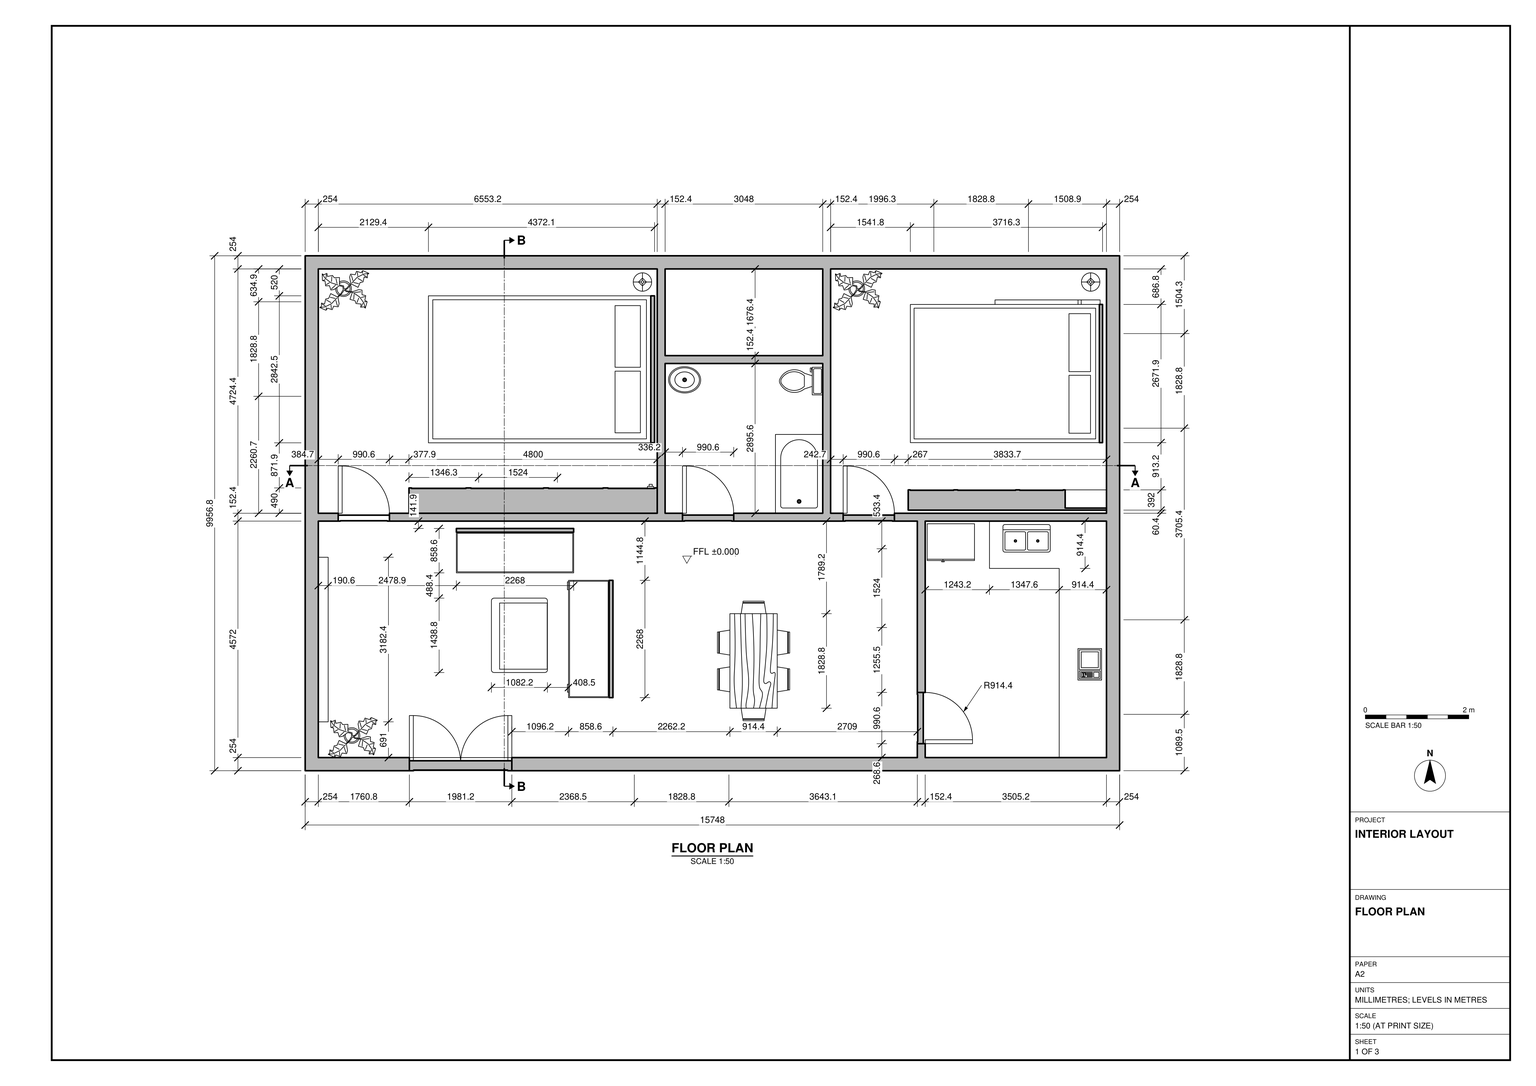
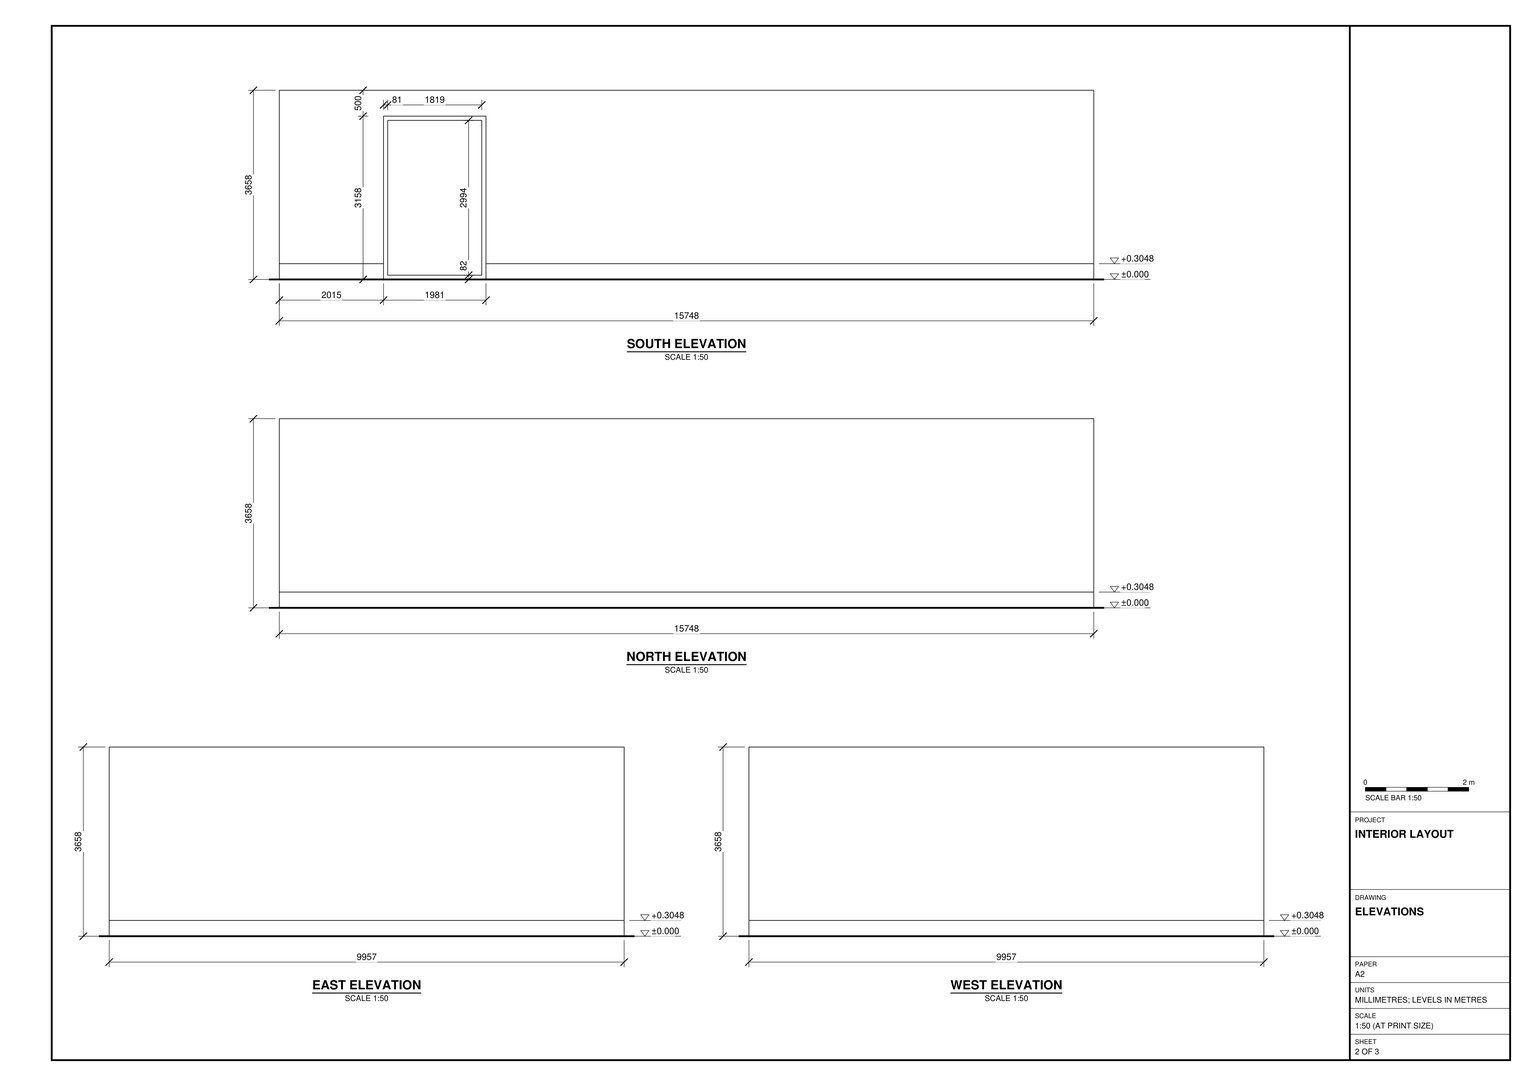
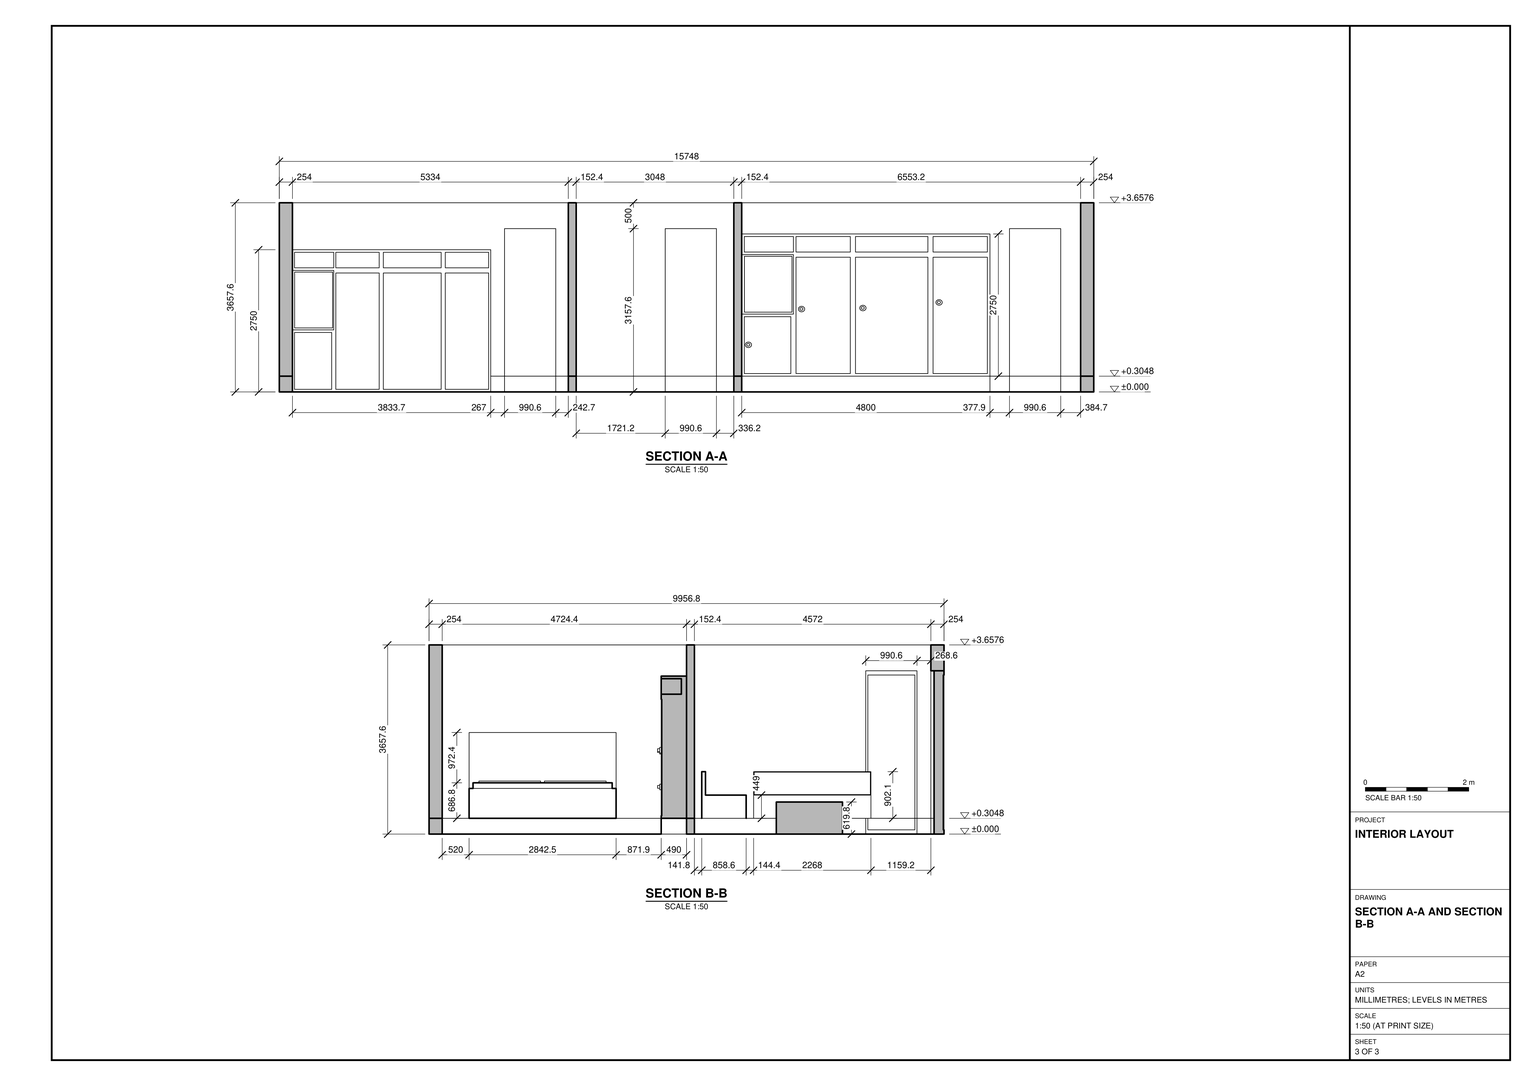
Build the interior in SketchUp using task_files/diagram_01.pdf. Work in millimetres. Use the floor plan to set out the rooms and the elevations and sections to establish heights. The rectangular shell measures 15748 mm east to west, 9956.8 mm north to south and 3657.6 mm high. Use a single ground-floor datum of 0 mm (±0.000). Model the floor base with the 304.8 mm base line shown in section, the 254 mm perimeter walls and the 152.4 mm partitions.

Place the bedrooms along the north side, with the bathroom between them and a separate enclosed space immediately north of the bathroom. Fit each bedroom with a bed and a built-in wardrobe along the south partition. Use section A-A for the wardrobe heights and front divisions, leaving room beside each wardrobe for the bedroom door. Place the basin, toilet and bathtub as shown in plan.

Set the double entrance door toward the west end of the south wall. Arrange the sofas and coffee table in the southwest living area, with the dining table and chairs between the seating and the enclosed southeast kitchen. Model the kitchen counter, double sink and appliances in their drawn positions. Decor and loose items such as plants, lamps and appliances may be any suitable library components.

Keep shell elements and individual furniture and joinery pieces in separate groups or components, and use components for repeated parts. Save one SketchUp model as output_files/furnished_two_bedroom_interior_with_built_in_wardrobes.skp.

# SketchUp Ruby script. Lengths in millimetres.
U = 1.mm
M = Sketchup.active_model
def pt(a) = Geom::Point3d.new(a.map { |v| v * U })
def face(e, loops, mat)
  f = e.add_face(loops[0].map { |a| pt(a) })
  loops[1..].each { |l| e.add_face(l.map { |a| pt(a) }).erase! }
  f.material = f.back_material = mat if mat
  f
end
# faces: each face lists its corners as indices into pts; further lists are holes
def faces(e, pts, list, mat = nil) = list.each { |f| face(e, (f[0].is_a?(Array) ? f : [f]).map { |l| l.map { |i| pts[i] } }, mat) }
# xy, xz, yz: faces in a plane at the given z, y or x. An outline is a flat list of corners, or four numbers for a rectangle; further outlines are holes
def ring(l) = l.size == 4 ? [[l[0], l[1]], [l[2], l[1]], [l[2], l[3]], [l[0], l[3]]] : l.each_slice(2).to_a
def flat(e, list, mat, &to3) = list.each { |f| face(e, (f[0].is_a?(Array) ? f : [f]).map { |l| ring(l).map { |u, v| to3.(u, v) } }, mat) }
def xy(e, z, list, mat = nil) = flat(e, list, mat) { |x, y| [x, y, z] }
def xz(e, y, list, mat = nil) = flat(e, list, mat) { |x, z| [x, y, z] }
def yz(e, x, list, mat = nil) = flat(e, list, mat) { |y, z| [x, y, z] }
def lines(e, pts, list) = list.each { |a, b| e.add_line(pt(pts[a]), pt(pts[b])) }
# prism: a flat outline (further loops are holes) pulled along v
def prism(e, loops, v, mat = nil)
  f = face(e, loops, mat); d = Geom::Vector3d.new(v.map { |x| x * U })
  f.pushpull(f.normal.samedirection?(d) ? d.length : -d.length)
end
def box(e, o, s, mat = nil) = prism(e, [[o, [o[0] + s[0], o[1], o[2]], [o[0] + s[0], o[1] + s[1], o[2]], [o[0], o[1] + s[1], o[2]]]], [0, 0, s[2]], mat)
def at(x, y, z, deg = 0) = Geom::Transformation.translation(pt([x, y, z])) * Geom::Transformation.rotation(ORIGIN, Z_AXIS, deg.degrees)
def axes(o, x, y, z) = Geom::Transformation.new([*x, 0, *y, 0, *z, 0, *pt(o).to_a, 1])
def part(name) = M.definitions.add(name)
# library, detail: a bought-in or finely detailed component or shape, given as its bounding box
def library(name, o, s) = part(name).tap { |d| box(d.entities, o, s) }
def detail(e, o, s) = box(e.add_group.entities, o, s)
def put(e, d, t, mat = nil) = e.add_instance(d, t).tap { |i| i.material = mat if mat }
def group(e, t, mat = nil) = e.add_group.tap { |g| g.transformation = t; g.material = mat if mat }.entities
root = M.entities
M.materials.add("[Carpet Pattern Squares Multi]").color = [138, 129, 101]
M.materials.add("[Color M08]").color = [30, 30, 30]
M.materials.add("[Color M09]").color = [0, 0, 0]
M.materials.add("[Leather Blue]").color = [45, 57, 74]
M.materials.add("[Mirror 02]").color = [229, 229, 229]
M.materials.add("[Translucent Glass Gray]").color = [128, 128, 128]
M.materials["[Translucent Glass Gray]"].alpha = 0.5
M.materials.add("[Wood Cherry Original]").color = [152, 86, 42]
M.materials.add("[Wood Veneer 01]").color = [120, 70, 37]
c1 = part("Framed panel")
xy(c1.entities,0,[[0,0,3940,620]],"[Wood Veneer 01]")
xy(c1.entities,161.4,[[161.4,0,3778.6,40]],"[Wood Veneer 01]")
xy(c1.entities,6068.6,[[161.4,0,3778.6,40]],"[Wood Veneer 01]")
xy(c1.entities,6230,[[0,0,3940,620]],"[Wood Veneer 01]")
xz(c1.entities,0,[[[0,0,3940,6230],[161.4,161.4,3778.6,6068.6]]],"[Wood Veneer 01]")
xz(c1.entities,40,[[161.4,161.4,3778.6,6068.6]],"[Wood Veneer 01]")
xz(c1.entities,620,[[0,0,3940,6230]],"[Wood Veneer 01]")
yz(c1.entities,0,[[0,0,620,6230]],"[Wood Veneer 01]")
yz(c1.entities,161.4,[[0,161.4,40,6068.6]],"[Wood Veneer 01]")
yz(c1.entities,3778.6,[[0,161.4,40,6068.6]],"[Wood Veneer 01]")
yz(c1.entities,3940,[[0,0,620,6230]],"[Wood Veneer 01]")
c2 = part("Component\#1")
xy(c2.entities,0,[[320,0,237.2,10.9,160,42.9,93.7,93.7,42.9,160,10.9,237.2,0,320,10.9,402.8,42.9,480,93.7,546.3,160,597.1,237.2,629.1,320,640,402.8,629.1,480,597.1,546.3,546.3,597.1,480,629.1,402.8,640,320,629.1,237.2,597.1,160,546.3,93.7,480,42.9,402.8,10.9]])
xy(c2.entities,230,[[[320,0,402.8,10.9,480,42.9,546.3,93.7,597.1,160,629.1,237.2,640,320,629.1,402.8,597.1,480,546.3,546.3,480,597.1,402.8,629.1,320,640,237.2,629.1,160,597.1,93.7,546.3,42.9,480,10.9,402.8,0,320,10.9,237.2,42.9,160,93.7,93.7,160,42.9,237.2,10.9],[322.3,149.9,281.5,158.6,244.3,177.6,213.2,205.6,190.5,240.7,177.6,280.4,175.5,322.1,184.2,363,203.2,400.2,231.2,431.2,266.2,453.9,305.9,466.8,347.7,468.9,388.5,460.2,425.7,441.2,456.7,413.2,479.5,378.2,492.3,338.5,494.5,296.8,485.8,255.9,466.8,218.7,438.8,187.7,403.8,165,364,152.1]]])
xy(c2.entities,470,[[322.3,149.9,364,152.1,403.8,165,438.8,187.7,466.8,218.7,485.8,255.9,494.5,296.8,492.3,338.5,479.5,378.2,456.7,413.2,425.7,441.2,388.5,460.2,347.7,468.9,305.9,466.8,266.2,453.9,231.2,431.2,203.2,400.2,184.2,363,175.5,322.1,177.6,280.4,190.5,240.7,213.2,205.6,244.3,177.6,281.5,158.6]])
p = [[237.2,10.9,0],[320,0,0],[320,0,230],[237.2,10.9,230],[402.8,10.9,0],[402.8,10.9,230],
  [160,42.9,0],[160,42.9,230],[480,42.9,0],[480,42.9,230],[93.7,93.7,0],[93.7,93.7,230],
  [546.3,93.7,0],[546.3,93.7,230],[42.9,160,0],[42.9,160,230],[597.1,160,0],[597.1,160,230],
  [10.9,237.2,0],[10.9,237.2,230],[629.1,237.2,0],[629.1,237.2,230],[0,320,0],[0,320,230],
  [640,320,0],[640,320,230],[10.9,402.8,0],[10.9,402.8,230],[629.1,402.8,0],[629.1,402.8,230],
  [42.9,480,0],[42.9,480,230],[597.1,480,0],[597.1,480,230],[93.7,546.3,0],[93.7,546.3,230],
  [546.3,546.3,0],[546.3,546.3,230],[160,597.1,0],[160,597.1,230],[480,597.1,0],[480,597.1,230],
  [237.2,629.1,0],[237.2,629.1,230],[402.8,629.1,0],[402.8,629.1,230],[320,640,0],[320,640,230],
  [281.5,158.6,230],[322.3,149.9,230],[322.3,149.9,470],[281.5,158.6,470],[364,152.1,230],[364,152.1,470],
  [403.8,165,230],[403.8,165,470],[244.3,177.6,230],[244.3,177.6,470],[438.8,187.7,230],[438.8,187.7,470],
  [213.2,205.6,230],[213.2,205.6,470],[466.8,218.7,230],[466.8,218.7,470],[190.5,240.7,230],[190.5,240.7,470],
  [485.8,255.9,230],[485.8,255.9,470],[177.6,280.4,230],[177.6,280.4,470],[494.5,296.8,230],[494.5,296.8,470],
  [175.5,322.1,230],[175.5,322.1,470],[492.3,338.5,230],[492.3,338.5,470],[184.2,363,230],[184.2,363,470],
  [479.5,378.2,230],[479.5,378.2,470],[203.2,400.2,230],[203.2,400.2,470],[456.7,413.2,230],[456.7,413.2,470],
  [231.2,431.2,230],[231.2,431.2,470],[425.7,441.2,230],[425.7,441.2,470],[266.2,453.9,230],[266.2,453.9,470],
  [388.5,460.2,230],[388.5,460.2,470],[305.9,466.8,230],[305.9,466.8,470],[347.7,468.9,230],[347.7,468.9,470]]
faces(c2.entities,p,[[0,1,2,3],[1,4,5,2],[6,0,3,7],[4,8,9,5],[10,6,7,11],[8,12,13,9],[14,10,11,15],[12,16,17,13],
  [18,14,15,19],[16,20,21,17],[22,18,19,23],[20,24,25,21],[26,22,23,27],[24,28,29,25],[30,26,27,31],[28,32,33,29],
  [34,30,31,35],[32,36,37,33],[38,34,35,39],[36,40,41,37],[42,38,39,43],[40,44,45,41],[46,42,43,47],[44,46,47,45],
  [48,49,50,51],[49,52,53,50],[52,54,55,53],[56,48,51,57],[54,58,59,55],[60,56,57,61],[58,62,63,59],[64,60,61,65],
  [62,66,67,63],[68,64,65,69],[66,70,71,67],[72,68,69,73],[70,74,75,71],[76,72,73,77],[74,78,79,75],[80,76,77,81],
  [78,82,83,79],[84,80,81,85],[82,86,87,83],[88,84,85,89],[86,90,91,87],[92,88,89,93],[90,94,95,91],[94,92,93,95]])
c3 = part("Bed frame")
xy(c3.entities,0,[[0,0,5267.6,3790]],"[Wood Veneer 01]")
xy(c3.entities,850,[[[0,0,5180,3790],[101.4,101.4,5078.6,3688.6]]],"[Wood Veneer 01]")
xy(c3.entities,1010,[[[101.4,101.4,5078.6,3688.6],[4347.5,257.5,4937.5,1847.5],[4347.5,1947.5,4937.5,3537.5]]],"[Leather Blue]")
xy(c3.entities,1060,[[4347.5,257.5,4937.5,1847.5],[4347.5,1947.5,4937.5,3537.5]])
xy(c3.entities,2440,[[5180,0,5267.6,3790]],"[Wood Veneer 01]")
xz(c3.entities,0,[[0,0,5267.6,0,5267.6,2440,5180,2440,5180,850,0,850]],"[Wood Veneer 01]")
xz(c3.entities,101.4,[[101.4,850,5078.6,1010]],"[Leather Blue]")
xz(c3.entities,257.5,[[4347.5,1010,4937.5,1060]])
xz(c3.entities,1847.5,[[4347.5,1010,4937.5,1060]])
xz(c3.entities,1947.5,[[4347.5,1010,4937.5,1060]])
xz(c3.entities,3537.5,[[4347.5,1010,4937.5,1060]])
xz(c3.entities,3688.6,[[101.4,850,5078.6,1010]],"[Leather Blue]")
xz(c3.entities,3790,[[0,0,0,850,5180,850,5180,2440,5267.6,2440,5267.6,0]],"[Wood Veneer 01]")
yz(c3.entities,0,[[0,0,3790,850]],"[Wood Veneer 01]")
yz(c3.entities,101.4,[[101.4,850,3688.6,1010]],"[Leather Blue]")
yz(c3.entities,4347.5,[[257.5,1010,1847.5,1060],[1947.5,1010,3537.5,1060]])
yz(c3.entities,4937.5,[[257.5,1010,1847.5,1060],[1947.5,1010,3537.5,1060]])
yz(c3.entities,5078.6,[[101.4,850,3688.6,1010]],"[Leather Blue]")
yz(c3.entities,5180,[[0,850,3790,2440]],"[Wood Veneer 01]")
yz(c3.entities,5267.6,[[0,0,3790,2440]],"[Wood Veneer 01]")
c4 = part("Component\#3")
xy(c4.entities,1000,[[[0,0,4320,1310],[33.6,33.6,4286.4,1276.4]],[33.6,33.6,4286.4,1276.4]])
xy(c4.entities,2010,[[0,1310,4320,1430]])
xz(c4.entities,0,[[0,0,4320,1000]])
xz(c4.entities,1310,[[[0,1000,4320,2010],[21.1,1021.1,4298.9,1988.9]],[21.1,1021.1,4298.9,1988.9]])
xz(c4.entities,1430,[[0,0,4320,2010]])
yz(c4.entities,0,[[0,0,0,1000,1310,1000,1310,2010,1430,2010,1430,0]])
yz(c4.entities,4320,[[0,0,1430,0,1430,2010,1310,2010,1310,1000,0,1000]])
c5 = library("floor plan.dwg",[0,0,0],[15748,9956.8,0.1])
c6 = part("Built-in wardrobe")
xy(c6.entities,304.8,[[2007.2,4978.4,6807.2,5468.4]])
xy(c6.entities,354.8,[[2057.2,5458.4,3107.2,5468.4],[3207.2,5458.4,4607.2,5468.4],[4707.2,5458.4,5757.2,5468.4],[5857.2,5458.4,6757.2,5468.4]],"[Wood Cherry Original]")
xy(c6.entities,1454.8,[[5857.2,5458.4,6757.2,5468.4]])
xy(c6.entities,1504.8,[[5807.2,5028.4,6807.2,5468.4]],"[Wood Cherry Original]")
xy(c6.entities,1542.2,[[5834.9,4988.4,6754.9,5028.4]],"[Color M09]")
xy(c6.entities,2604.8,[[2057.2,5458.4,3107.2,5468.4],[3207.2,5458.4,4607.2,5468.4],[4707.2,5458.4,5757.2,5468.4]],"[Wood Cherry Original]")
xy(c6.entities,2622.2,[[5834.9,4988.4,6754.9,5028.4]],"[Color M09]")
xy(c6.entities,2654.8,[[5807.2,5028.4,6807.2,5468.4]],"[Wood Cherry Original]")
xy(c6.entities,2704.8,[[2057.2,5078.4,3107.2,5468.4],[3207.2,5078.4,4607.2,5468.4],[4707.2,5078.4,5757.2,5468.4],[5807.2,5078.4,6757.2,5468.4]])
xy(c6.entities,3004.8,[[2057.2,5078.4,3107.2,5468.4],[3207.2,5078.4,4607.2,5468.4],[4707.2,5078.4,5757.2,5468.4],[5807.2,5078.4,6757.2,5468.4]])
xy(c6.entities,3054.8,[[2007.2,4978.4,6807.2,5468.4]],"[Wood Cherry Original]")
xz(c6.entities,4978.4,[[2007.2,304.8,6807.2,3054.8]])
xz(c6.entities,4988.4,[[5834.9,1542.2,6754.9,2622.2]],"[Mirror 02]")
xz(c6.entities,5028.4,[[[5807.2,1504.8,6807.2,2654.8],[5834.9,1542.2,6754.9,2622.2]]],"[Color M09]")
xz(c6.entities,5078.4,[[2057.2,2704.8,3107.2,3004.8],[3207.2,2704.8,4607.2,3004.8],[4707.2,2704.8,5757.2,3004.8],[5807.2,2704.8,6757.2,3004.8]])
xz(c6.entities,5458.4,[[2057.2,354.8,3107.2,2604.8],[3207.2,354.8,4607.2,2604.8],[4707.2,354.8,5757.2,2604.8],[5857.2,354.8,6757.2,1454.8]],"[Wood Cherry Original]")
xz(c6.entities,5468.4,[[2057.2,2704.8,3107.2,3004.8],[3207.2,2704.8,4607.2,3004.8],[4707.2,2704.8,5757.2,3004.8],[5807.2,2704.8,6757.2,3004.8]],"[Translucent Glass Gray]")
xz(c6.entities,5468.4,[[[2007.2,304.8,2007.2,3054.8,6807.2,3054.8,6807.2,2654.8,5807.2,2654.8,5807.2,1504.8,6807.2,1504.8,6807.2,304.8],[3207.2,354.8,4607.2,2604.8],[2057.2,354.8,3107.2,2604.8],[4707.2,354.8,5757.2,2604.8],[5857.2,354.8,6757.2,1454.8],[3207.2,2704.8,4607.2,3004.8],[2057.2,2704.8,3107.2,3004.8],[4707.2,2704.8,5757.2,3004.8],[5807.2,2704.8,6757.2,3004.8]]],"[Wood Cherry Original]")
yz(c6.entities,2007.2,[[4978.4,304.8,5468.4,3054.8]],"[Wood Cherry Original]")
yz(c6.entities,2057.2,[[5458.4,354.8,5468.4,2604.8]],"[Wood Cherry Original]")
yz(c6.entities,3107.2,[[5078.4,2704.8,5468.4,3004.8]])
yz(c6.entities,3107.2,[[5458.4,354.8,5468.4,2604.8]],"[Wood Cherry Original]")
yz(c6.entities,3207.2,[[5078.4,2704.8,5468.4,3004.8]])
yz(c6.entities,3207.2,[[5458.4,354.8,5468.4,2604.8]],"[Wood Cherry Original]")
yz(c6.entities,4607.2,[[5078.4,2704.8,5468.4,3004.8]])
yz(c6.entities,4607.2,[[5458.4,354.8,5468.4,2604.8]],"[Wood Cherry Original]")
yz(c6.entities,4707.2,[[5078.4,2704.8,5468.4,3004.8]])
yz(c6.entities,4707.2,[[5458.4,354.8,5468.4,2604.8]],"[Wood Cherry Original]")
yz(c6.entities,5757.2,[[5458.4,354.8,5468.4,1504.8],[5078.4,2704.8,5468.4,3004.8]])
yz(c6.entities,5757.2,[[5458.4,1504.8,5468.4,2604.8]],"[Wood Cherry Original]")
yz(c6.entities,5807.2,[[5078.4,2704.8,5468.4,3004.8]])
yz(c6.entities,5807.2,[[5028.4,1504.8,5468.4,2654.8]],"[Wood Cherry Original]")
yz(c6.entities,5834.9,[[4988.4,1542.2,5028.4,2622.2]],"[Color M09]")
yz(c6.entities,5857.2,[[5458.4,354.8,5468.4,1454.8]],"[Wood Cherry Original]")
yz(c6.entities,6754.9,[[4988.4,1542.2,5028.4,2622.2]],"[Color M09]")
yz(c6.entities,6757.2,[[5458.4,354.8,5468.4,1454.8],[5078.4,2704.8,5468.4,3004.8]])
yz(c6.entities,6807.2,[[4978.4,304.8,4978.4,3054.8,5468.4,3054.8,5468.4,2654.8,5028.4,2654.8,5028.4,1504.8,5468.4,1504.8,5468.4,304.8]])
c7 = part("Two-bedroom interior")
put(c7.entities,c2,axes([4983.2,6404.2,1676],[0.19072,0,0],[0,0,-0.1675],[0,0.17,0]),"[Color M08]")
put(c7.entities,c2,axes([3510.2,6404.2,1784.6],[0.19072,0,0],[0,0,-0.1675],[0,0.17,0]),"[Color M08]")
put(c7.entities,c2,axes([7197,6404.2,964.7],[0.19072,0,0],[0,0,-0.1675],[0,0.17,0]),"[Color M08]")
put(c7.entities,c3,axes([2963.3,7286.1,304.8],[0.83,0,0],[0,0.75,0],[0,0,0.68]))
put(c7.entities,c4,axes([3503.4,4771.4,304.8],[0.525,0,0],[0,0.6004,0],[0,0,0.4488]),"[Wood Cherry Original]")
put(c7.entities,c3,axes([12281.8,7289.9,0],[0.7055,0,0],[0,0.705,0],[0,0,0.68]))
put(c7.entities,c5,at(579.9,945.8,304.8))
put(c7.entities,c6,axes([10637.1,2001.9,-304.8],[0.79869,0,0],[0,0.8,0],[0,0,1]))
put(c7.entities,c4,axes([5672.1,4627,304.8],[0,-0.525,0],[0.6004,0,0],[0,0,0.4488]),"[Wood Cherry Original]")
put(c7.entities,c2,axes([6169.2,6404.3,1656.1],[0.19072,0,0],[0,0,-0.1675],[0,0.17,0]),"[Color M08]")
g1 = group(c7.entities,at(579.9,945.8,0))
xy(g1,0,[[0,0,0,9956.8,15748,9956.8,15748,0,3996,0,3996,254,15494,254,15494,9702.8,254,9702.8,254,254,2014.8,254,2014.8,0],[2014.8,0,3996,254],[254,254,11836.4,254,11836.4,522.6,11988.8,522.6,11988.8,254,15494,254,15494,4826,11988.8,4826,11988.8,1513.2,11836.4,1513.2,11836.4,4826,11393.3,4826,11393.3,4978.4,15494,4978.4,15494,9702.8,10160,9702.8,10160,4978.4,10402.7,4978.4,10402.7,4826,8286.4,4826,8286.4,4978.4,10007.6,4978.4,10007.6,7874,6959.6,7874,6959.6,4978.4,7295.8,4978.4,7295.8,4826,1629.3,4826,1629.3,4978.4,2007.2,4978.4,2007.2,5468.4,6807.2,5468.4,6807.2,9702.8,254,9702.8,254,4978.4,638.7,4978.4,638.7,4826,254,4826],[11836.4,254,11988.8,522.6],[11836.4,1513.2,11836.4,4826,11393.3,4826,11393.3,4978.4,15494,4978.4,15494,4826,11988.8,4826,11988.8,1513.2],
  [254,4826,638.7,4978.4],[1629.3,4826,1629.3,4978.4,6807.2,4978.4,6807.2,9702.8,6959.6,9702.8,6959.6,8026.4,10007.6,8026.4,10007.6,9702.8,10160,9702.8,10160,4978.4,10007.6,4978.4,10007.6,7874,6959.6,7874,6959.6,4978.4,7295.8,4978.4,7295.8,4826],[6959.6,8026.4,10007.6,9702.8]])
xy(g1,304.8,[[[0,0,2014.8,0,2014.8,254,254,254,254,4826,638.7,4826,638.7,4978.4,254,4978.4,254,9702.8,6807.2,9702.8,6807.2,4978.4,1629.3,4978.4,1629.3,4826,7295.8,4826,7295.8,4978.4,6959.6,4978.4,6959.6,7874,10007.6,7874,10007.6,4978.4,10160,4978.4,10160,9702.8,15494,9702.8,15494,4978.4,11393.3,4978.4,11393.3,4826,11836.4,4826,11836.4,1513.2,11988.8,1513.2,11988.8,4826,15494,4826,15494,254,11988.8,254,11988.8,522.6,11836.4,522.6,11836.4,254,3996,254,3996,0,15748,0,15748,9956.8,0,9956.8],[6959.6,8026.4,10007.6,9702.8]],[2007.2,4978.4,6807.2,5468.4],[6959.6,8026.4,10007.6,9702.8]])
xy(g1,354.8,[[2057.2,5458.4,3107.2,5468.4],[3207.2,5458.4,4607.2,5468.4],[4707.2,5458.4,5757.2,5468.4],[5857.2,5458.4,6757.2,5468.4]],"[Wood Cherry Original]")
xy(g1,1454.8,[[5857.2,5458.4,6757.2,5468.4]])
xy(g1,1504.8,[[5807.2,5028.4,6807.2,5468.4]],"[Wood Cherry Original]")
xy(g1,1542.2,[[5834.9,4988.4,6754.9,5028.4]],"[Color M09]")
xy(g1,2604.8,[[2057.2,5458.4,3107.2,5468.4],[3207.2,5458.4,4607.2,5468.4],[4707.2,5458.4,5757.2,5468.4]],"[Wood Cherry Original]")
xy(g1,2622.2,[[5834.9,4988.4,6754.9,5028.4]],"[Color M09]")
xy(g1,2654.8,[[5807.2,5028.4,6807.2,5468.4]],"[Wood Cherry Original]")
xy(g1,2704.8,[[2057.2,5078.4,3107.2,5468.4],[3207.2,5078.4,4607.2,5468.4],[4707.2,5078.4,5757.2,5468.4],[5807.2,5078.4,6757.2,5468.4]])
xy(g1,3004.8,[[2057.2,5078.4,3107.2,5468.4],[3207.2,5078.4,4607.2,5468.4],[4707.2,5078.4,5757.2,5468.4],[5807.2,5078.4,6757.2,5468.4]])
xy(g1,3054.8,[[2007.2,4978.4,6807.2,5468.4]],"[Wood Cherry Original]")
xy(g1,3157.6,[[2014.8,0,3996,254],[11836.4,522.6,11988.8,1513.2],[638.7,4826,1629.3,4978.4],[7295.8,4826,8286.4,4978.4],[10402.7,4826,11393.3,4978.4]])
xy(g1,3657.6,[[[0,0,15748,9956.8],[254,254,11836.4,4826],[254,4978.4,6807.2,9702.8],[10160,4978.4,15494,9702.8],[11988.8,254,15494,4826],[6959.6,4978.4,10007.6,9702.8]]])
xy(g1,3657.6,[[6959.6,7874,10007.6,8026.4]],"[Translucent Glass Gray]")
xz(g1,0,[[0,0,2014.8,304.8],[3996,0,15748,304.8],[0,304.8,0,3657.6,15748,3657.6,15748,304.8,3996,304.8,3996,3157.6,2014.8,3157.6,2014.8,304.8]])
xz(g1,254,[[254,0,2014.8,304.8],[3996,0,11836.4,304.8],[11988.8,0,15494,304.8],[254,304.8,2014.8,304.8,2014.8,3157.6,3996,3157.6,3996,304.8,11836.4,304.8,11836.4,3657.6,254,3657.6],[11988.8,304.8,15494,3657.6]])
xz(g1,522.6,[[11836.4,0,11988.8,304.8],[11836.4,304.8,11988.8,3157.6]])
xz(g1,1513.2,[[11836.4,0,11988.8,304.8],[11836.4,304.8,11988.8,3157.6]])
xz(g1,4826,[[254,0,638.7,304.8],[8286.4,0,8286.4,3157.6,7295.8,3157.6,7295.8,304.8,1629.3,304.8,1629.3,3157.6,638.7,3157.6,638.7,304.8,254,304.8,254,3657.6,11836.4,3657.6,11836.4,304.8,11393.3,304.8,11393.3,3157.6,10402.7,3157.6,10402.7,0],[1629.3,0,7295.8,304.8],[11393.3,0,11836.4,304.8],[11988.8,0,15494,304.8],
  [11988.8,304.8,15494,3657.6]])
xz(g1,4978.4,[[254,0,638.7,304.8],[1629.3,0,2007.2,304.8],[2007.2,0,6807.2,304.8],[6959.6,0,7295.8,304.8],[8286.4,0,8286.4,3157.6,7295.8,3157.6,7295.8,304.8,6959.6,304.8,6959.6,3657.6,10007.6,3657.6,10007.6,0],
  [10007.6,0,10160,304.8],[10160,0,10402.7,0,10402.7,3157.6,11393.3,3157.6,11393.3,304.8,15494,304.8,15494,3657.6,10160,3657.6],[11393.3,0,15494,304.8],[254,304.8,638.7,304.8,638.7,3157.6,1629.3,3157.6,1629.3,304.8,2007.2,304.8,2007.2,3054.8,6807.2,3054.8,6807.2,3657.6,254,3657.6],[2007.2,304.8,6807.2,3054.8]])
xz(g1,4988.4,[[5834.9,1542.2,6754.9,2622.2]],"[Mirror 02]")
xz(g1,5028.4,[[[5807.2,1504.8,6807.2,2654.8],[5834.9,1542.2,6754.9,2622.2]]],"[Color M09]")
xz(g1,5078.4,[[2057.2,2704.8,3107.2,3004.8],[3207.2,2704.8,4607.2,3004.8],[4707.2,2704.8,5757.2,3004.8],[5807.2,2704.8,6757.2,3004.8]])
xz(g1,5458.4,[[2057.2,354.8,3107.2,2604.8],[3207.2,354.8,4607.2,2604.8],[4707.2,354.8,5757.2,2604.8],[5857.2,354.8,6757.2,1454.8]],"[Wood Cherry Original]")
xz(g1,5468.4,[[2007.2,0,6807.2,304.8]])
xz(g1,5468.4,[[2057.2,2704.8,3107.2,3004.8],[3207.2,2704.8,4607.2,3004.8],[4707.2,2704.8,5757.2,3004.8],[5807.2,2704.8,6757.2,3004.8]],"[Translucent Glass Gray]")
xz(g1,5468.4,[[[2007.2,304.8,2007.2,3054.8,6807.2,3054.8,6807.2,2654.8,5807.2,2654.8,5807.2,1504.8,6807.2,1504.8,6807.2,304.8],[3207.2,354.8,4607.2,2604.8],[4707.2,354.8,5757.2,2604.8],[2057.2,354.8,3107.2,2604.8],[5857.2,354.8,6757.2,1454.8],[3207.2,2704.8,4607.2,3004.8],[4707.2,2704.8,5757.2,3004.8],[2057.2,2704.8,3107.2,3004.8],[5807.2,2704.8,6757.2,3004.8]]],"[Wood Cherry Original]")
xz(g1,7874,[[6959.6,0,10007.6,304.8]])
xz(g1,7874,[[6959.6,304.8,10007.6,3657.6]],"[Translucent Glass Gray]")
xz(g1,8026.4,[[6959.6,0,10007.6,304.8]])
xz(g1,8026.4,[[6959.6,304.8,10007.6,3657.6]],"[Translucent Glass Gray]")
xz(g1,9702.8,[[254,0,6807.2,304.8],[6959.6,0,10007.6,304.8],[10160,0,15494,304.8],[254,304.8,6807.2,3657.6],[6959.6,304.8,10007.6,3657.6],
  [10160,304.8,15494,3657.6]])
xz(g1,9956.8,[[0,0,15748,3657.6]])
yz(g1,0,[[0,0,9956.8,3657.6]])
yz(g1,254,[[254,0,4826,304.8],[4978.4,0,9702.8,304.8],[254,304.8,4826,3657.6],[4978.4,304.8,9702.8,3657.6]])
yz(g1,638.7,[[4826,0,4978.4,304.8],[4826,304.8,4978.4,3157.6]])
yz(g1,1629.3,[[4826,0,4978.4,304.8],[4826,304.8,4978.4,3157.6]])
yz(g1,2007.2,[[4978.4,0,5468.4,304.8]])
yz(g1,2007.2,[[4978.4,304.8,5468.4,3054.8]],"[Wood Cherry Original]")
yz(g1,2014.8,[[0,0,254,304.8],[0,304.8,254,3157.6]])
yz(g1,2057.2,[[5078.4,2704.8,5468.4,3004.8]])
yz(g1,2057.2,[[5458.4,354.8,5468.4,2604.8]],"[Wood Cherry Original]")
yz(g1,3107.2,[[5078.4,2704.8,5468.4,3004.8]])
yz(g1,3107.2,[[5458.4,354.8,5468.4,2604.8]],"[Wood Cherry Original]")
yz(g1,3207.2,[[5078.4,2704.8,5468.4,3004.8]])
yz(g1,3207.2,[[5458.4,354.8,5468.4,2604.8]],"[Wood Cherry Original]")
yz(g1,3996,[[0,0,254,304.8],[0,304.8,254,3157.6]])
yz(g1,4607.2,[[5078.4,2704.8,5468.4,3004.8]])
yz(g1,4607.2,[[5458.4,354.8,5468.4,2604.8]],"[Wood Cherry Original]")
yz(g1,4707.2,[[5078.4,2704.8,5468.4,3004.8]])
yz(g1,4707.2,[[5458.4,354.8,5468.4,2604.8]],"[Wood Cherry Original]")
yz(g1,5757.2,[[5458.4,354.8,5468.4,1504.8],[5078.4,2704.8,5468.4,3004.8]])
yz(g1,5757.2,[[5458.4,1504.8,5468.4,2604.8]],"[Wood Cherry Original]")
yz(g1,5807.2,[[5078.4,2704.8,5468.4,3004.8]])
yz(g1,5807.2,[[5028.4,1504.8,5468.4,2654.8]],"[Wood Cherry Original]")
yz(g1,5834.9,[[4988.4,1542.2,5028.4,2622.2]],"[Color M09]")
yz(g1,5857.2,[[5458.4,354.8,5468.4,1454.8]],"[Wood Cherry Original]")
yz(g1,6754.9,[[4988.4,1542.2,5028.4,2622.2]],"[Color M09]")
yz(g1,6757.2,[[5458.4,354.8,5468.4,1454.8],[5078.4,2704.8,5468.4,3004.8]])
yz(g1,6807.2,[[4978.4,0,5468.4,304.8],[5468.4,0,9702.8,304.8],[4978.4,304.8,4978.4,3054.8,5468.4,3054.8,5468.4,2654.8,5028.4,2654.8,5028.4,1504.8,5468.4,1504.8,5468.4,304.8],[5468.4,304.8,9702.8,304.8,9702.8,3657.6,4978.4,3657.6,4978.4,3054.8,5468.4,3054.8,5468.4,2654.8,5028.4,2654.8,5028.4,1504.8,5468.4,1504.8]])
yz(g1,6959.6,[[4978.4,0,7874,304.8],[8026.4,0,9702.8,304.8],[4978.4,304.8,7874,3657.6],[8026.4,304.8,9702.8,3657.6]])
yz(g1,7295.8,[[4826,0,4978.4,304.8],[4826,304.8,4978.4,3157.6]])
yz(g1,8286.4,[[4826,0,4978.4,3157.6]])
yz(g1,10007.6,[[4978.4,0,7874,304.8],[8026.4,0,9702.8,304.8],[4978.4,304.8,7874,3657.6],[8026.4,304.8,9702.8,3657.6]])
yz(g1,10160,[[4978.4,0,9702.8,304.8],[4978.4,304.8,9702.8,3657.6]])
yz(g1,10402.7,[[4826,0,4978.4,3157.6]])
yz(g1,11393.3,[[4826,0,4978.4,304.8],[4826,304.8,4978.4,3157.6]])
yz(g1,11836.4,[[254,0,522.6,304.8],[1513.2,0,4826,304.8],[254,304.8,522.6,304.8,522.6,3157.6,1513.2,3157.6,1513.2,304.8,4826,304.8,4826,3657.6,254,3657.6]])
yz(g1,11988.8,[[254,0,522.6,304.8],[1513.2,0,4826,304.8],[254,304.8,254,3657.6,4826,3657.6,4826,304.8,1513.2,304.8,1513.2,3157.6,522.6,3157.6,522.6,304.8]])
yz(g1,15494,[[254,0,4826,304.8],[4978.4,0,9702.8,304.8],[254,304.8,4826,3657.6],[4978.4,304.8,9702.8,3657.6]])
yz(g1,15748,[[0,0,9956.8,3657.6]])
xy(root,-304.8,[[3759.4,1962.7,4679.4,3242.7]])
xy(root,315.2,[[3759.4,1962.7,4679.4,3242.7]],"[Carpet Pattern Squares Multi]")
xz(root,1962.7,[[3759.4,-304.8,4679.4,315.2]])
xz(root,3242.7,[[3759.4,-304.8,4679.4,315.2]])
yz(root,3759.4,[[1962.7,-304.8,3242.7,315.2]])
yz(root,4679.4,[[1962.7,-304.8,3242.7,315.2]])
p = [[1629.3,4978.4,2852.8],[1629.3,4826,2852.8]]
lines(root,p,[[0,1]])
put(root,c1,axes([2014.8,0,-304.8],[0.50284,0,0],[0,0.31,0],[0,0,0.50684]))
put(root,c7,at(-579.9,-945.8,-304.8))
put(root,c1,axes([7295.8,4826,-304.8],[0.25142,0,0],[0,0.1891,0],[0,0,0.50684]))
put(root,c1,axes([11836.4,1513.2,-304.8],[0,-0.25142,0],[0.186,0,0],[0,0,0.50684]))
put(root,c1,axes([638.7,4826,-304.8],[0.25142,0,0],[0,0.186,0],[0,0,0.50684]))
put(root,c1,axes([10402.7,4826,-304.8],[0.25142,0,0],[0,0.1891,0],[0,0,0.50684]))
